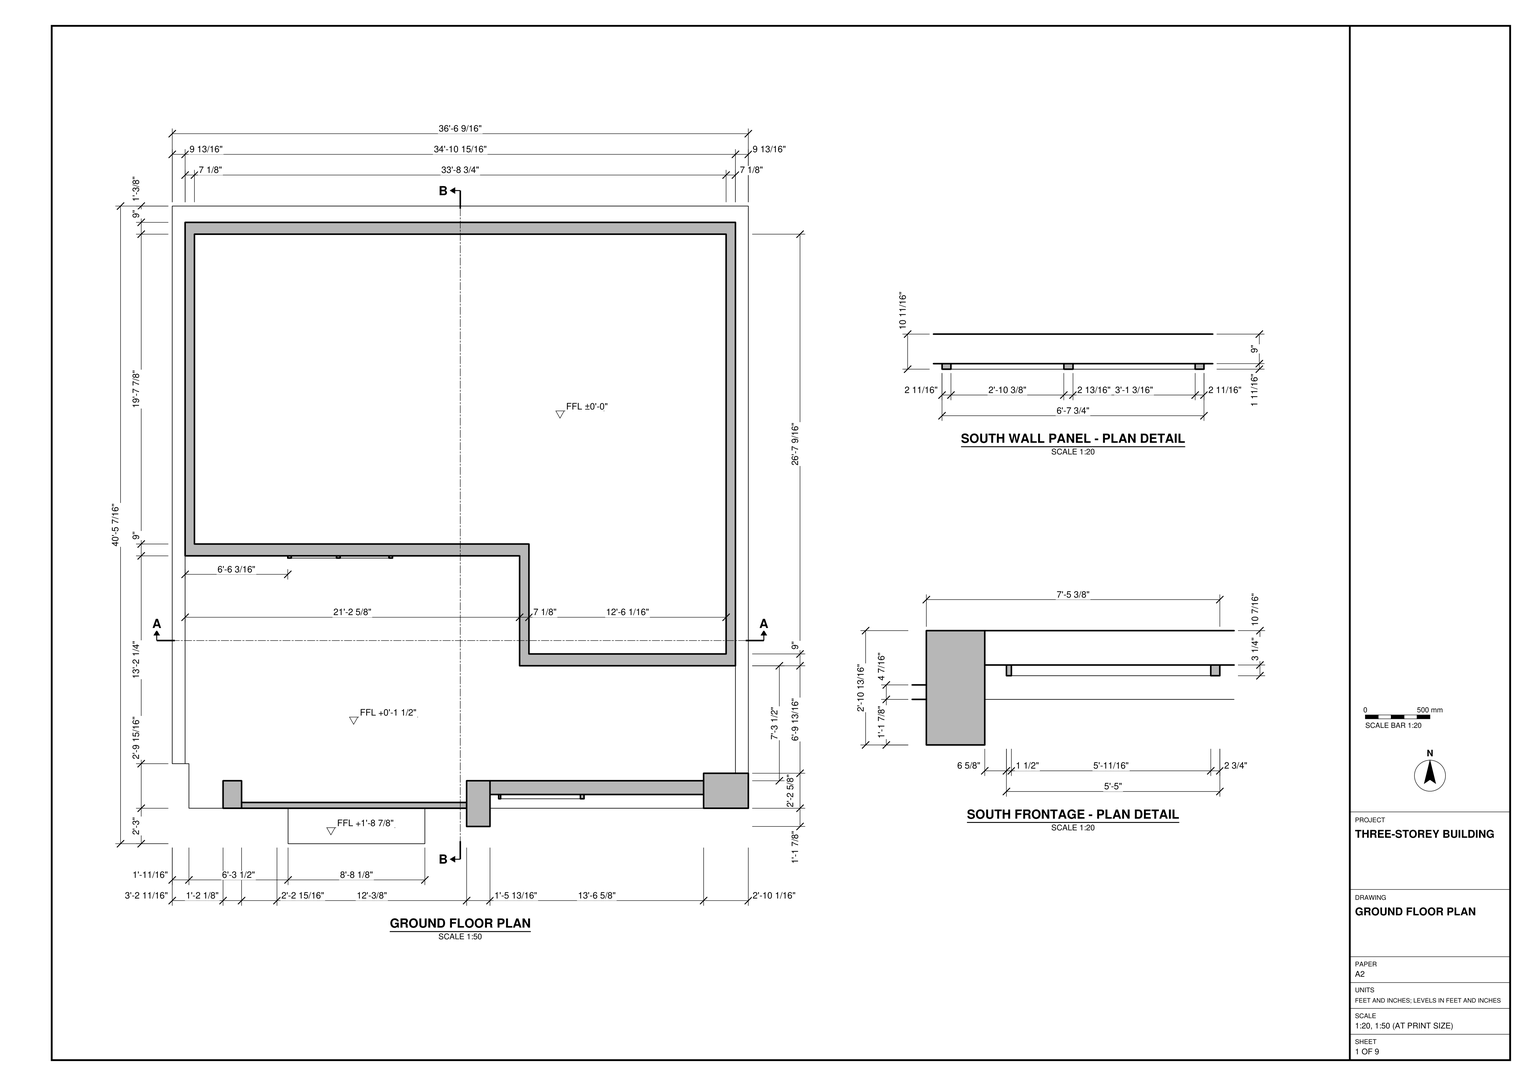
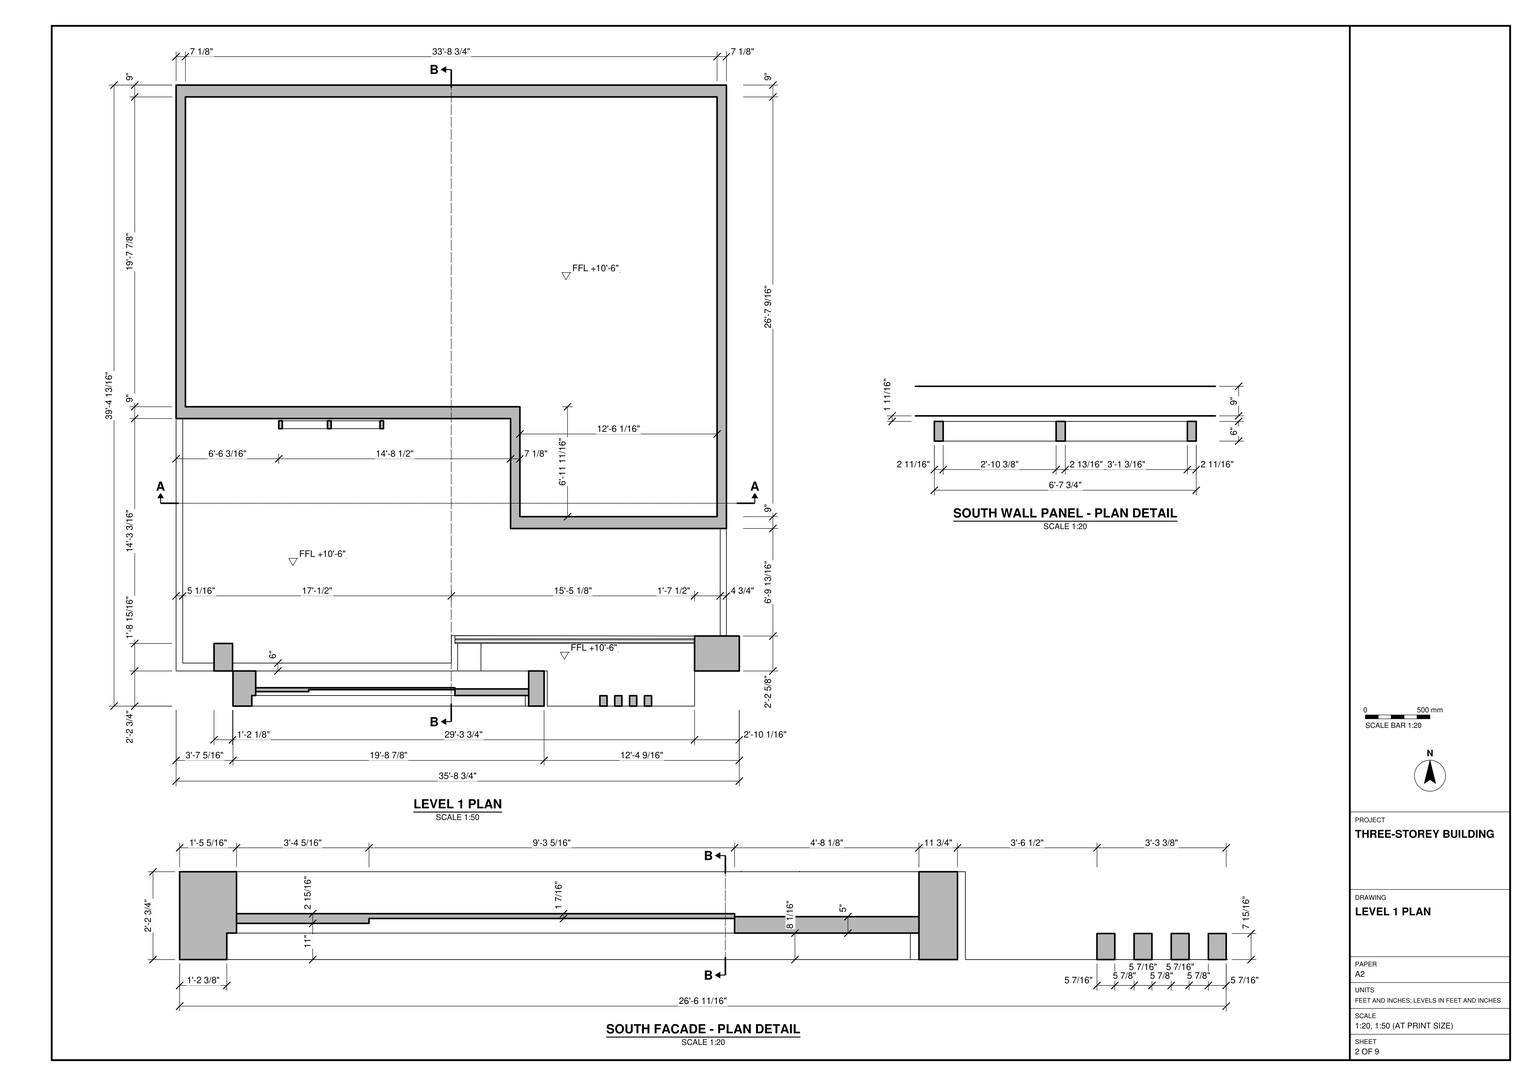
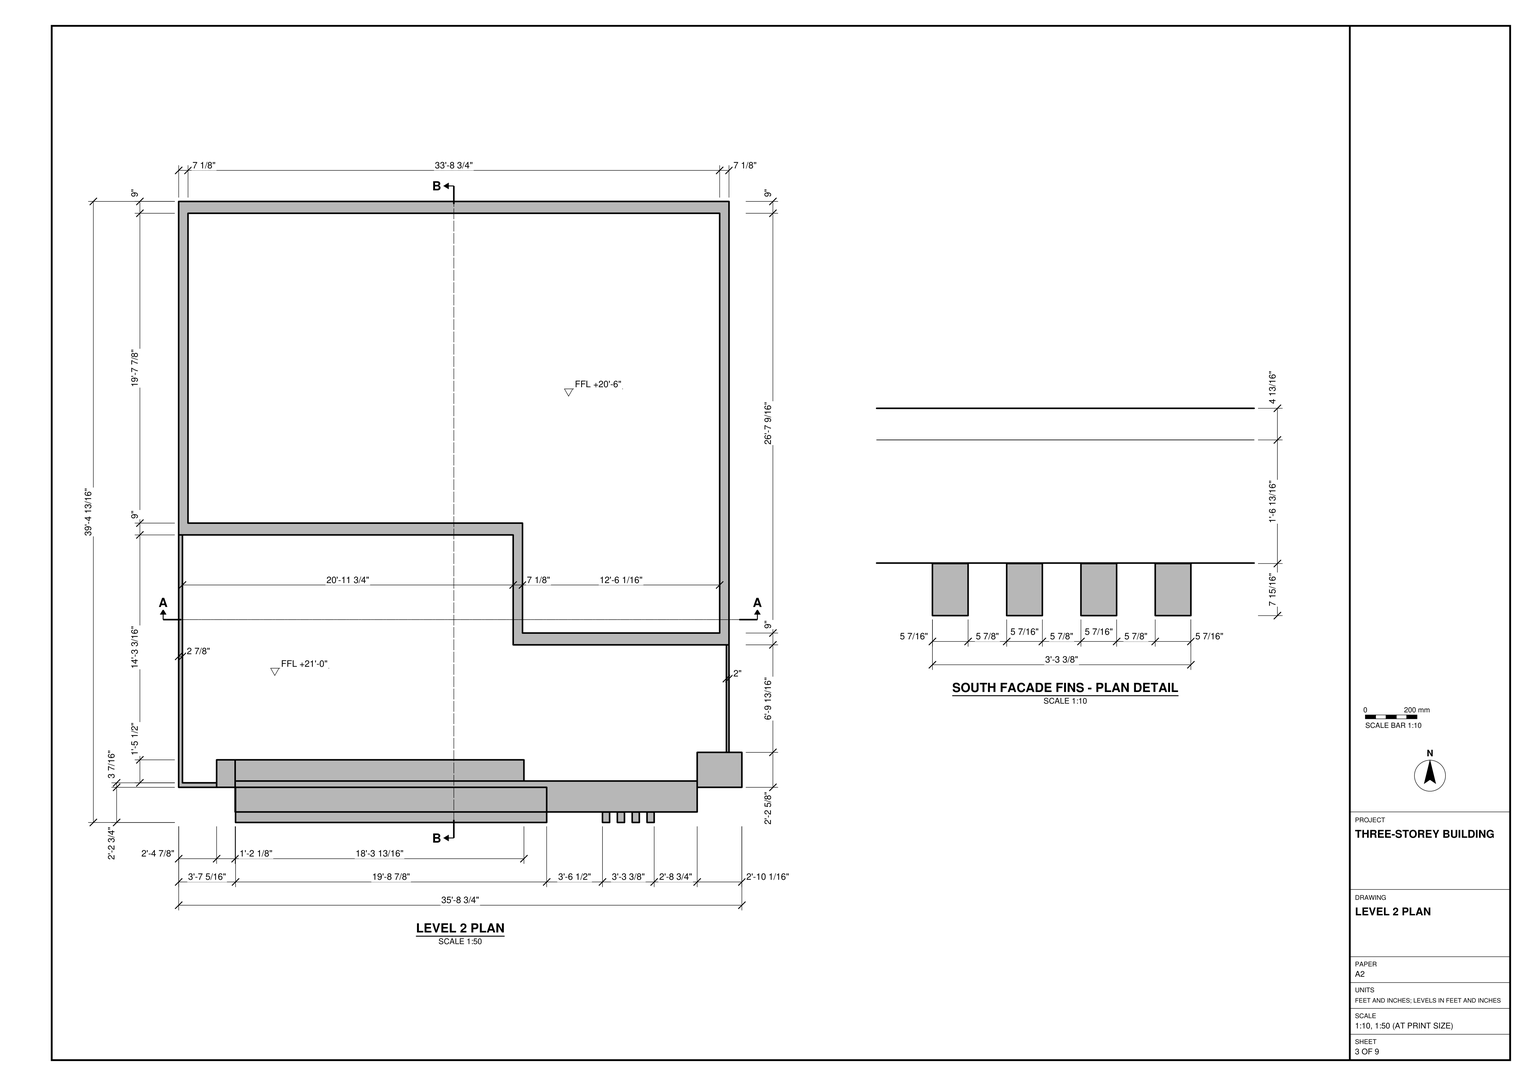
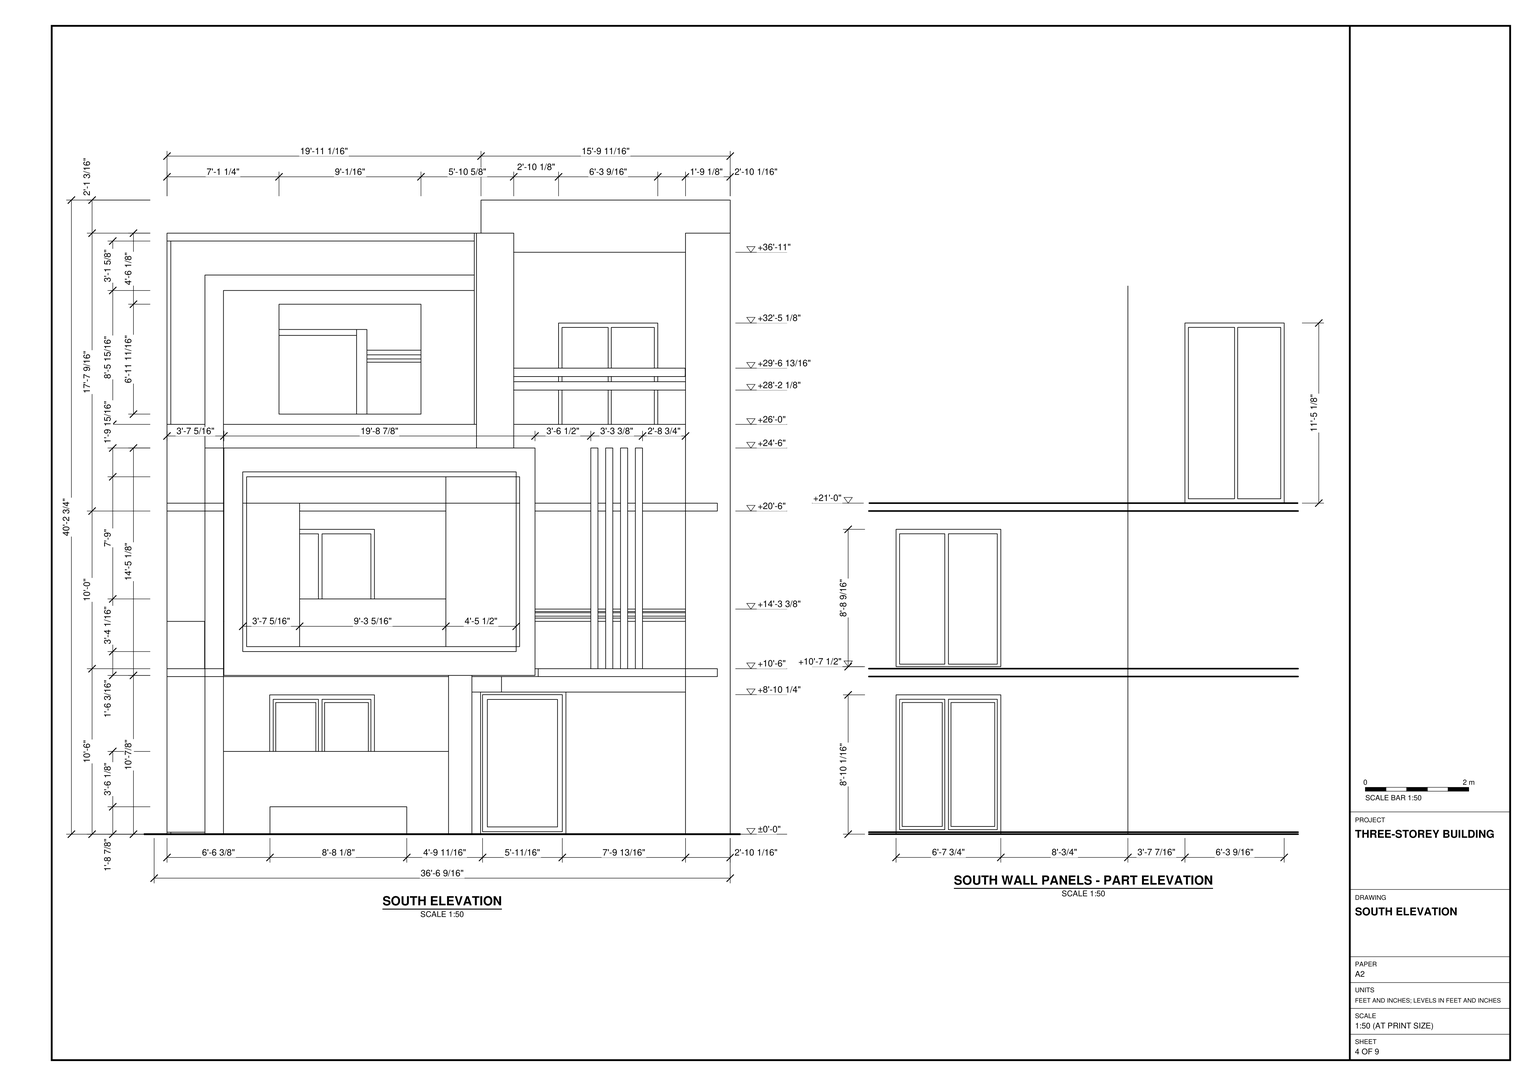
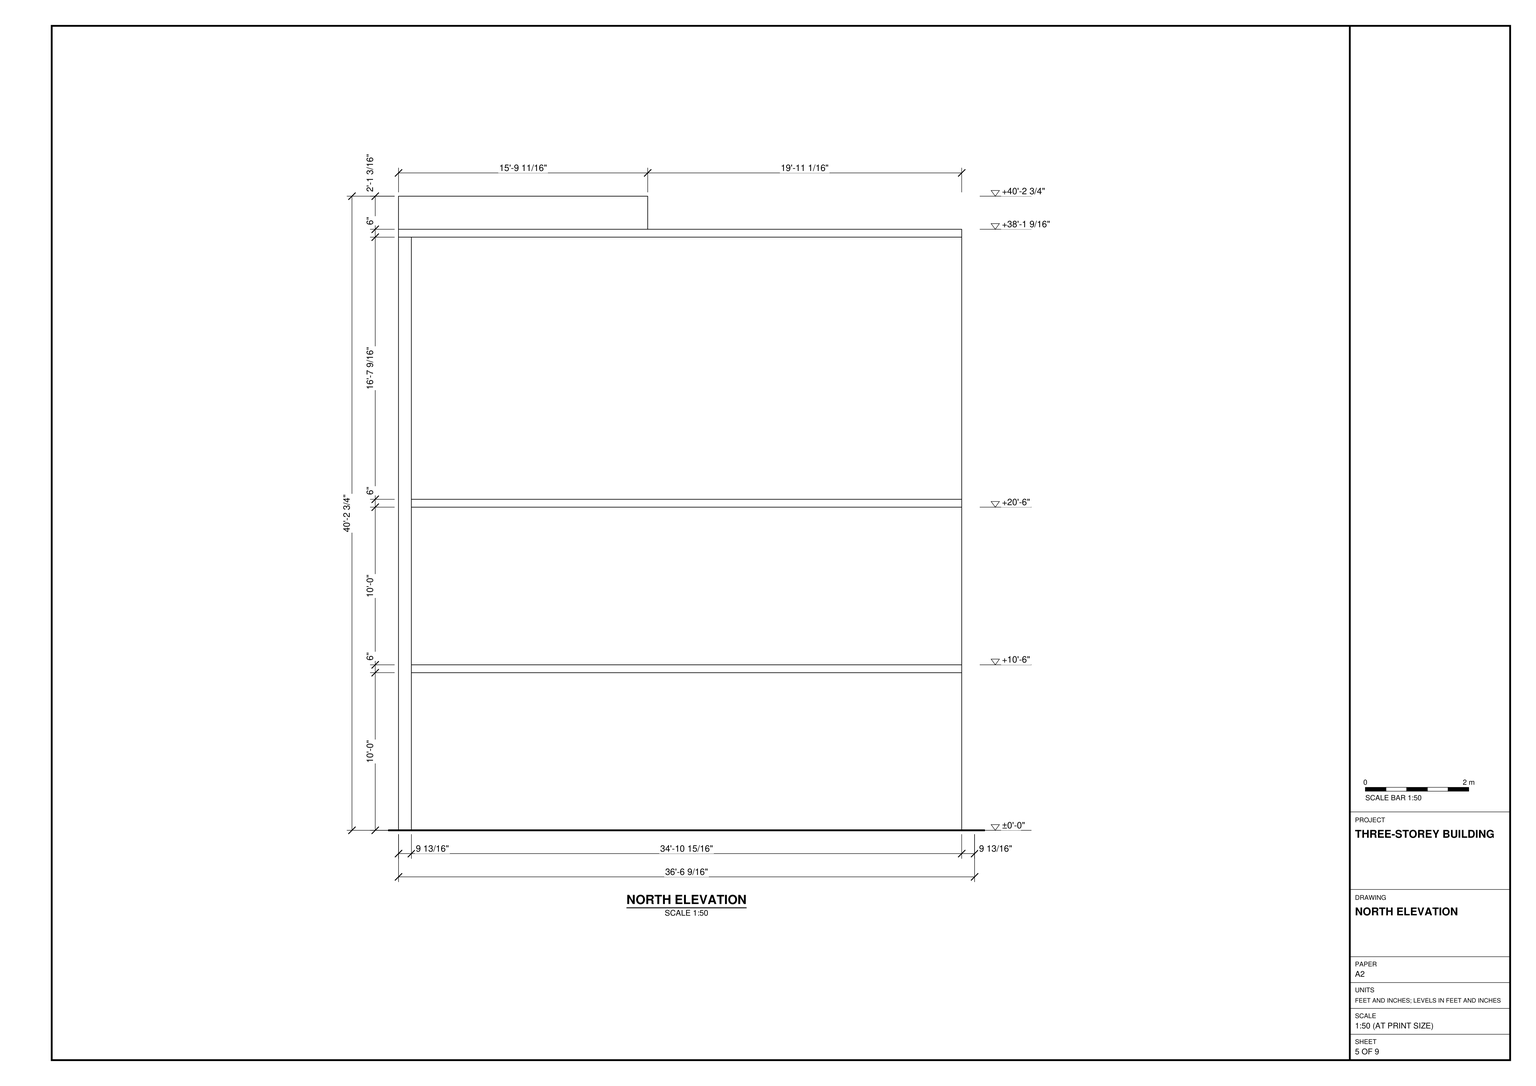
Build the three-storey building in SketchUp from task_files/diagram_01.pdf. Work in feet and inches. Set the overall width along X to 36'-6 9/16", depth along Y to 40'-5 7/16", and height along Z to 40'-2 3/4". Use finished floor levels of ±0'-0", +10'-6", and +20'-6" relative to the ground floor.

Lay out the enclosed part of each storey with a straight north wall and a stepped south wall. The east bay extends farther south than the west bay, leaving a deeper open area in front of the west bay. Use the wall thicknesses dimensioned in plan, including 9" for the east–west walls and 7 1/8" for the north–south returns. Model the floor slabs, the changes in floor height at the frontage, and the roof profile shown in the sections and elevations.

Use the enlarged plans to locate the panels on the recessed south wall and to set out the frontage piers, openings, projecting horizontal members, and closely spaced fins. Follow the drawings for any stairs, built-in joinery, and main furniture rather than adding an interior layout. Keep walls, slabs, the roof, and each furniture or joinery piece in separate groups or components; use components for repeated parts. Any decor or loose items shown may be represented by suitable library components. Save one SketchUp model as output_files/three_storey_building_with_a_stepped_south_frontage.skp.

# SketchUp Ruby script. Lengths in inches.
U = 1.inch
M = Sketchup.active_model
def pt(a) = Geom::Point3d.new(a.map { |v| v * U })
def face(e, loops, mat)
  f = e.add_face(loops[0].map { |a| pt(a) })
  loops[1..].each { |l| e.add_face(l.map { |a| pt(a) }).erase! }
  f.material = f.back_material = mat if mat
  f
end
# faces: each face lists its corners as indices into pts; further lists are holes
def faces(e, pts, list, mat = nil) = list.each { |f| face(e, (f[0].is_a?(Array) ? f : [f]).map { |l| l.map { |i| pts[i] } }, mat) }
# xy, xz, yz: faces in a plane at the given z, y or x. An outline is a flat list of corners, or four numbers for a rectangle; further outlines are holes
def ring(l) = l.size == 4 ? [[l[0], l[1]], [l[2], l[1]], [l[2], l[3]], [l[0], l[3]]] : l.each_slice(2).to_a
def flat(e, list, mat, &to3) = list.each { |f| face(e, (f[0].is_a?(Array) ? f : [f]).map { |l| ring(l).map { |u, v| to3.(u, v) } }, mat) }
def xy(e, z, list, mat = nil) = flat(e, list, mat) { |x, y| [x, y, z] }
def xz(e, y, list, mat = nil) = flat(e, list, mat) { |x, z| [x, y, z] }
def yz(e, x, list, mat = nil) = flat(e, list, mat) { |y, z| [x, y, z] }
def lines(e, pts, list) = list.each { |a, b| e.add_line(pt(pts[a]), pt(pts[b])) }
# prism: a flat outline (further loops are holes) pulled along v
def prism(e, loops, v, mat = nil)
  f = face(e, loops, mat); d = Geom::Vector3d.new(v.map { |x| x * U })
  f.pushpull(f.normal.samedirection?(d) ? d.length : -d.length)
end
def box(e, o, s, mat = nil) = prism(e, [[o, [o[0] + s[0], o[1], o[2]], [o[0] + s[0], o[1] + s[1], o[2]], [o[0], o[1] + s[1], o[2]]]], [0, 0, s[2]], mat)
def at(x, y, z, deg = 0) = Geom::Transformation.translation(pt([x, y, z])) * Geom::Transformation.rotation(ORIGIN, Z_AXIS, deg.degrees)
def axes(o, x, y, z) = Geom::Transformation.new([*x, 0, *y, 0, *z, 0, *pt(o).to_a, 1])
def part(name) = M.definitions.add(name)
# library, detail: a bought-in or finely detailed component or shape, given as its bounding box
def library(name, o, s) = part(name).tap { |d| box(d.entities, o, s) }
def detail(e, o, s) = box(e.add_group.entities, o, s)
def put(e, d, t, mat = nil) = e.add_instance(d, t).tap { |i| i.material = mat if mat }
def group(e, t, mat = nil) = e.add_group.tap { |g| g.transformation = t; g.material = mat if mat }.entities
root = M.entities
g1 = group(root,at(0,0,0))
prism(g1,[[[87.96,211.47,232.0625],[87.96,211.47,127.5],[167.7,211.47,127.5],[167.7,211.47,232.0625]],[[165.02,211.47,129.4],[127.83,211.47,129.4],[127.83,211.47,228.66],[165.02,211.47,228.66]],[[125.05,211.47,228.66],[125.05,211.47,129.4],[90.65,211.47,129.4],[90.65,211.47,228.66]]],[0,6,0])
xy(g1,0,[[88.19,0,192.32,27],[224.11,13.125,241.9,47.9375],[12.71,27,12.71,60.9375,9.8,60.9375,9.8,219.16,87.96,219.16,87.96,217.47,167.7,217.47,167.7,219.16,264.44,219.16,264.44,135.47,428.75,135.47,428.75,53.625,404.52,53.625,404.52,47.9375,224.11,47.9375,224.11,31.41,52.79,31.41,52.79,47.9375,38.69,47.9375,38.69,27],[38.69,27,52.79,47.9375],[52.79,27,79.73,31.41],
  [79.73,27,88.19,31.41],[88.19,27,192.32,31.41],[192.32,27,224.11,31.41],[241.9,27,404.52,27,404.52,37.47,313.48,37.47,313.48,34.22,248.5,34.22,248.5,37.47,241.9,37.47],[248.5,34.22,313.48,37.47],
  [241.9,37.47,404.52,47.9375],[428.75,53.625,438.55,53.625,438.55,485.4375,0,485.4375,0,60.9375,9.8,60.9375,9.8,473.03,428.75,473.03],[[264.44,135.47,264.44,219.16,9.8,219.16,9.8,473.03,428.75,473.03,428.75,135.47],[271.55,144.47,421.64,144.47,421.64,464.03,16.91,464.03,16.91,228.16,271.55,228.16]],[271.55,144.47,421.64,144.47,421.64,464.03,16.91,464.03,16.91,228.16,271.55,228.16],[87.96,217.47,167.7,219.16]])
xy(g1,1.5,[[12.71,27,38.69,27,38.69,47.9375,52.79,47.9375,52.79,31.41,224.11,31.41,224.11,47.9375,404.52,47.9375,404.52,53.625,428.75,53.625,428.75,135.47,264.44,135.47,264.44,219.16,167.7,219.16,167.7,217.47,87.96,217.47,87.96,219.16,9.8,219.16,9.8,60.9375,12.71,60.9375]])
xy(g1,1.9,[[250.01,34.22,310.72,37.47]])
xy(g1,3.4,[[90.65,217.47,125.05,219.16],[127.83,217.47,165.02,219.16]])
xy(g1,20.875,[[88.19,0,192.32,27]])
xy(g1,63,[[52.79,27,224.11,31.41]])
xy(g1,102.66,[[90.65,217.47,125.05,219.16],[127.83,217.47,165.02,219.16]])
xy(g1,106.0625,[[87.96,217.47,167.7,219.16]])
xy(g1,106.22,[[250.01,34.22,310.72,37.47]])
xy(g1,108.1875,[[248.5,34.22,313.48,37.47],[241.9,37.47,404.52,47.9375]])
xy(g1,120,[[292.36,0.25,292.36,27,264.44,27,264.44,47.9375,428.75,47.9375,428.75,27,404.52,27,404.52,0.25],[9.8,27,9.8,219.16,264.44,219.16,264.44,47.9375,224.11,47.9375,224.11,27,79.73,27,79.73,47.9375,26.8125,47.9375,26.8125,60.9375,12.71,60.9375,12.71,27],[12.71,27,26.8125,60.9375],[26.8125,27,79.73,47.9375],[241.9,27,264.44,47.9375],
  [264.44,47.9375,428.75,135.47],[[264.44,135.47,264.44,219.16,9.8,219.16,9.8,473.03,428.75,473.03,428.75,135.47],[271.55,144.47,421.64,144.47,421.64,464.03,16.91,464.03,16.91,228.16,271.55,228.16]]])
xy(g1,126,[[292.36,0.25,332.43,0.25,332.43,8.18,337.86,8.18,337.86,0.25,343.73,0.25,343.73,8.18,349.16,8.18,349.16,0.25,355.04,0.25,355.04,8.18,360.47,8.18,360.47,0.25,366.35,0.25,366.35,8.18,371.78,8.18,371.78,0.25,404.52,0.25,404.52,47.9375,241.9,47.9375,241.9,27,292.36,27],[332.43,0.25,337.86,8.18],[343.73,0.25,349.16,8.18],[355.04,0.25,360.47,8.18],[366.35,0.25,371.78,8.18],
  [224.11,13.125,241.9,47.9375],[9.8,27,9.8,219.16,14.85,219.16,14.85,33,38.46,33,38.46,27],[38.46,27,52.79,27,52.79,33,219.37,33,219.37,53.9375,404.52,53.625,404.52,47.9375,428.75,47.9375,428.75,53.9375,424.01,53.9375,424.01,135.47,264.44,135.47,264.44,219.16,14.85,219.16,14.85,33,38.46,33],[52.79,27,52.79,33,219.37,33,219.37,53.9375,404.52,53.625,404.52,47.9375,224.11,47.9375,224.11,27],[404.52,27,428.75,47.9375],
  [424.01,53.9375,428.75,135.47],[[264.44,135.47,264.44,219.16,9.8,219.16,9.8,473.03,428.75,473.03,428.75,135.47],[271.55,144.47,421.64,144.47,421.64,464.03,16.91,464.03,16.91,228.16,271.55,228.16]],[271.55,144.47,421.64,144.47,421.64,464.03,16.91,464.03,16.91,228.16,271.55,228.16]])
xy(g1,162,[[9.8,27,38.46,27,38.46,33,14.85,33,14.85,219.16,9.8,219.16],[52.79,27,224.11,27,224.11,47.9375,222.08,47.9375,222.08,53.81,297.83,53.81,219.37,53.9375,219.37,33,52.79,33],[222.08,47.9375,222.08,53.81,297.83,53.81,404.52,53.625,404.52,47.9375],[424.01,53.9375,428.75,135.47]])
xy(g1,164.5,[[222.08,47.9375,404.52,47.9375,404.52,53.625,297.83,53.81,222.08,53.81]])
xy(g1,246,[[9.8,27,264.44,60.9375],[264.44,27,428.75,135.47],[9.8,60.9375,264.44,219.16],[[264.44,135.47,264.44,219.16,9.8,219.16,9.8,473.03,428.75,473.03,428.75,135.47],[271.55,144.47,421.64,144.47,421.64,464.03,16.91,464.03,16.91,228.16,271.55,228.16]],[271.55,144.47,421.64,144.47,421.64,464.03,16.91,464.03,16.91,228.16,271.55,228.16]])
xy(g1,252,[[52.79,8.25,404.52,27],[9.8,27,9.8,219.16,12.6875,219.16,12.6875,30.4375,38.69,30.4375,38.69,27],[38.69,27,52.79,27,52.79,47.9375,272.63,47.9375,272.63,31.8125,404.52,31.8125,404.52,27,428.75,27,428.75,53.625,426.77,53.625,426.77,135.47,264.44,135.47,264.44,219.16,12.6875,219.16,12.6875,30.4375,38.69,30.4375],[52.79,27,404.52,31.8125],[426.77,53.625,428.75,135.47],
  [[264.44,135.47,264.44,219.16,9.8,219.16,9.8,473.03,428.75,473.03,428.75,135.47],[271.55,144.47,421.64,144.47,421.64,464.03,16.91,464.03,16.91,228.16,271.55,228.16]]])
xy(g1,294,[[245.41,0.25,269.66,8.25],[269.66,0.25,273.76,8.25],[332.43,0.25,337.86,8.18],[343.73,0.25,349.16,8.18],[355.04,0.25,360.47,8.18],
  [366.35,0.25,371.78,8.18]])
xy(g1,312,[[52.79,8.25,245.41,8.25,243.73,31.8125,52.79,31.8125],[273.76,8.25,404.52,8.25,404.52,31.8125,272.08,31.8125],[9.8,27,38.69,27,38.69,30.4375,12.6875,30.4375,12.6875,219.16,9.8,219.16],[426.77,53.625,428.75,135.47]])
xy(g1,319.8,[[95.0625,31.8125,154.12,47.9375],[154.12,31.8125,161.99,47.9375],[161.99,31.8125,203.14,47.9375]])
xy(g1,358,[[38.69,31.8125,52.79,47.9375]])
xy(g1,379.72,[[95.0625,31.8125,154.12,47.9375]])
xy(g1,384.23,[[95.0625,31.8125,154.12,47.9375],[154.12,31.8125,161.99,47.9375]])
xy(g1,403.46,[[95.0625,31.8125,203.14,47.9375]])
xy(g1,413.92,[[52.79,27,243.73,31.8125]])
xy(g1,425.6875,[[38.69,27,243.73,27,243.73,31.8125,272.63,31.8125,272.63,47.9375,38.69,47.9375]])
xy(g1,443,[[248.84,31.8125,248.84,170.625,260.46,170.625,260.46,42.72,404.52,42.72,404.52,31.8125]])
xy(g1,451.5625,[[404.52,31.8125,426.77,53.625],[426.77,31.8125,428.75,53.625],[428.75,31.8125,438.55,53.625],[260.46,42.72,260.46,135.47,426.77,135.47,426.77,53.625,404.52,53.625,404.52,42.72],[426.77,53.625,428.75,135.47],
  [428.75,53.625,438.55,473.03],[[264.44,135.47,264.44,219.16,9.8,219.16,9.8,473.03,428.75,473.03,428.75,135.47],[271.55,144.47,421.64,144.47,421.64,464.03,16.91,464.03,16.91,228.16,271.55,228.16]],[260.46,135.47,260.46,170.625,248.84,170.625,248.84,219.16,264.44,219.16,264.44,135.47],[9.8,161.41,248.84,219.16]])
xy(g1,457.5625,[[245.41,0.25,273.76,0.25,273.76,8.25,272.08,31.8125,243.73,31.8125,245.41,8.25],[404.52,27,438.55,31.8125],[248.84,41.51,438.55,41.51,438.55,473.03,9.8,473.03,9.8,161.41,248.84,161.41]])
xy(g1,482.75,[[248.84,31.8125,438.55,41.51]])
xz(g1,0,[[88.19,0,192.32,20.875]])
xz(g1,0.25,[[292.36,120,404.52,126],[332.43,126,337.86,294],[343.73,126,349.16,294],[355.04,126,360.47,294],[366.35,126,371.78,294],
  [245.41,294,273.76,457.5625]])
xz(g1,8.18,[[332.43,126,337.86,294],[343.73,126,349.16,294],[355.04,126,360.47,294],[366.35,126,371.78,294]])
xz(g1,8.25,[[52.79,252,404.52,252,404.52,312,273.76,312,273.76,294,245.41,294,245.41,312,52.79,312]])
xz(g1,13.125,[[224.11,0,241.9,126]])
xz(g1,27,[[12.71,0,38.69,1.5],[38.69,0,52.79,120],[52.79,0,88.19,0,88.19,20.875,192.32,20.875,192.32,0,224.11,0,224.11,63,52.79,63],[88.19,0,192.32,20.875],[404.52,0,438.55,0,438.55,457.5625,404.52,457.5625,404.52,252,428.75,252,428.75,246,404.52,246,404.52,126,428.75,126,428.75,120,404.52,120],
  [9.8,120,26.8125,126],[26.8125,120,38.69,126],[38.69,120,52.79,126],[52.79,120,224.11,126],[241.9,120,292.36,126],
  [404.52,120,428.75,126],[9.8,126,38.46,162],[38.69,126,52.79,246],[52.79,126,224.11,162],[9.8,246,38.69,252],
  [38.69,246,52.79,252],[52.79,246,404.52,252],[404.52,246,428.75,252],[9.8,252,38.69,312],[38.69,252,52.79,294],
  [38.69,294,52.79,294,52.79,413.92,243.73,413.92,243.73,425.6875,38.69,425.6875]])
xz(g1,30.4375,[[12.6875,252,38.69,312]])
xz(g1,31.41,[[52.79,0,79.73,1.5],[79.73,0,88.19,1.5],[88.19,0,192.32,1.5],[192.32,0,224.11,1.5],[52.79,1.5,224.11,63]])
xz(g1,31.8125,[[52.79,252,272.63,312],[272.63,252,404.52,312],[[52.79,312,243.73,413.92],[95.0625,319.8,203.14,403.46]],[243.73,312,272.08,425.6875],[272.08,312,272.63,425.6875],
  [154.12,319.8,161.99,384.23],[95.0625,379.72,154.12,384.23],[243.73,425.6875,243.73,457.5625,248.84,457.5625,248.84,443,272.08,443,272.08,425.6875],[248.84,443,272.08,457.5625],[272.08,443,404.52,443,404.52,457.5625,438.55,457.5625,438.55,482.75,248.84,482.75,248.84,457.5625,272.08,457.5625],
  [404.52,451.5625,426.77,457.5625],[426.77,451.5625,428.75,457.5625]])
xz(g1,33,[[14.85,126,38.46,162],[52.79,126,219.37,162]])
xz(g1,34.22,[[[248.5,0,313.48,108.1875],[250.01,1.9,310.72,106.22]]])
xz(g1,37.47,[[241.9,0,248.5,108.1875],[[248.5,0,313.48,108.1875],[250.01,1.9,310.72,106.22]],[313.48,0,404.52,108.1875],[[250.01,1.9,310.72,106.22],[253.65,5.55,307.08,102.58]],[253.65,5.55,307.08,102.58]])
xz(g1,41.51,[[248.84,457.5625,438.55,482.75]])
xz(g1,42.72,[[260.46,443,404.52,451.5625]])
xz(g1,47.9375,[[38.69,0,52.79,1.5],[224.11,0,241.9,1.5],[241.9,0,404.52,1.5],[38.69,1.5,52.79,120],[224.11,1.5,241.9,120],
  [241.9,1.5,404.52,108.1875],[38.69,120,52.79,126],[224.11,120,241.9,126],[241.9,120,428.75,126],[38.69,126,52.79,358],
  [224.11,126,404.52,162],[222.08,162,404.52,164.5],[[52.79,252,52.79,358,38.69,358,38.69,425.6875,272.63,425.6875,272.63,252],[95.0625,319.8,203.14,403.46]],[154.12,319.8,161.99,384.23],[95.0625,379.72,154.12,384.23]])
xz(g1,53.625,[[404.52,0,428.75,1.5],[[428.75,0,428.75,1.5,404.52,1.5,404.52,451.5625,438.55,451.5625,438.55,0],[426.77,252,428.75,312]],[426.77,252,428.75,312]])
xz(g1,53.81,[[222.08,162,297.83,164.5]])
xz(g1,53.9375,[[424.01,126,428.75,162]])
xz(g1,60.9375,[[9.8,0,12.71,1.5]])
xz(g1,135.47,[[264.44,0,428.75,1.5],[264.44,1.5,428.75,120],[264.44,120,428.75,126],[264.44,126,424.01,126,424.01,162,428.75,162,428.75,246,264.44,246],[424.01,126,428.75,162],
  [264.44,246,428.75,252],[264.44,252,307.87,252,307.87,389.125,383.41,389.125,383.41,252,426.77,252,426.77,451.5625,264.44,451.5625],[[307.87,252,383.41,389.125],[310.5,255.33,345.64,385.8],[348.02,255.33,380.78,385.8]],[426.77,252,428.75,312],[310.5,255.33,345.64,385.8],
  [348.02,255.33,380.78,385.8],[426.77,312,428.75,451.5625]])
xz(g1,144.47,[[271.55,0,421.64,120],[271.55,120,421.64,126],[271.55,126,421.64,246],[271.55,246,421.64,252],[271.55,252,421.64,451.5625]])
xz(g1,161.41,[[9.8,451.5625,248.84,457.5625]])
xz(g1,170.625,[[248.84,443,260.46,451.5625]])
xz(g1,217.47,[[87.96,0,167.7,1.5],[[87.96,1.5,167.7,106.0625],[127.83,3.4,165.02,102.66],[90.65,3.4,125.05,102.66]]])
xz(g1,219.16,[[9.8,0,87.96,1.5],[[87.96,0,167.7,106.0625],[127.83,3.4,165.02,102.66],[90.65,3.4,125.05,102.66]],[167.7,0,264.44,1.5],[9.8,1.5,87.96,1.5,87.96,106.0625,167.7,106.0625,167.7,1.5,264.44,1.5,264.44,120,9.8,120],[[90.65,3.4,125.05,102.66],[92.59,5.85,123.11,100.21]],
  [[127.83,3.4,165.02,102.66],[129.77,5.85,163.08,100.21]],[92.59,5.85,123.11,100.21],[129.77,5.85,163.08,100.21],[9.8,120,264.44,126],[14.85,126,264.44,126,264.44,246,9.8,246,9.8,162,14.85,162],
  [9.8,126,14.85,162],[9.8,246,264.44,252],[9.8,252,12.6875,312],[12.6875,252,264.44,451.5625],[9.8,312,12.6875,451.5625]])
xz(g1,228.16,[[16.91,0,271.55,120],[16.91,120,271.55,126],[16.91,126,271.55,246],[16.91,246,271.55,252],[16.91,252,271.55,451.5625]])
xz(g1,464.03,[[16.91,0,421.64,120],[16.91,120,421.64,126],[16.91,126,421.64,246],[16.91,246,421.64,252],[16.91,252,421.64,451.5625]])
xz(g1,473.03,[[9.8,0,428.75,120],[9.8,120,428.75,126],[9.8,126,428.75,246],[9.8,246,428.75,252],[9.8,252,428.75,451.5625],
  [9.8,451.5625,438.55,457.5625]])
yz(g1,9.8,[[60.9375,0,219.16,1.5],[219.16,0,473.03,120],[27,120,219.16,126],[219.16,120,473.03,126],[27,126,219.16,162],
  [219.16,126,473.03,246],[27,246,219.16,252],[219.16,246,473.03,252],[27,252,219.16,312],[219.16,252,473.03,451.5625],
  [161.41,451.5625,473.03,457.5625]])
yz(g1,12.6875,[[30.4375,252,219.16,312]])
yz(g1,12.71,[[27,0,60.9375,1.5]])
yz(g1,14.85,[[33,126,219.16,162]])
yz(g1,16.91,[[228.16,0,464.03,120],[228.16,120,464.03,126],[228.16,126,464.03,246],[228.16,246,464.03,252],[228.16,252,464.03,451.5625]])
yz(g1,38.46,[[27,126,33,162]])
yz(g1,38.69,[[27,0,47.9375,1.5],[27,1.5,27,252,30.4375,252,30.4375,425.6875,31.8125,425.6875,31.8125,358,47.9375,358,47.9375,1.5],[27,252,30.4375,312],[27,312,30.4375,425.6875],[31.8125,358,47.9375,425.6875]])
yz(g1,52.79,[[27,0,31.41,63],[31.41,0,47.9375,1.5],[31.41,1.5,47.9375,1.5,47.9375,126,27,126,27,63,31.41,63],[27,126,33,162],[33,126,47.9375,126,47.9375,252,27,252,27,162,33,162],
  [8.25,252,27,294],[27,252,31.8125,312],[31.8125,252,47.9375,358],[8.25,294,27,312],[27,312,31.8125,413.92]])
yz(g1,87.96,[[217.47,0,219.16,1.5],[217.47,1.5,219.16,106.0625]])
yz(g1,88.19,[[0,0,27,20.875]])
yz(g1,90.65,[[217.47,3.4,219.16,102.66]])
yz(g1,95.0625,[[31.8125,319.8,47.9375,379.72],[31.8125,379.72,47.9375,384.23],[31.8125,384.23,47.9375,403.46]])
yz(g1,125.05,[[217.47,3.4,219.16,102.66]])
yz(g1,127.83,[[217.47,3.4,219.16,102.66]])
yz(g1,154.12,[[31.8125,319.8,47.9375,379.72],[31.8125,379.72,47.9375,384.23]])
yz(g1,161.99,[[[31.8125,319.8,47.9375,384.23],[36.6,364.95,36.15,365.01,35.73,365.18,35.37,365.46,35.09,365.82,34.91,366.24,34.85,366.7,34.91,367.15,35.09,367.57,35.37,367.94,35.73,368.21,36.15,368.39,36.6,368.45,37.06,368.39,37.48,368.21,37.84,367.94,38.12,367.57,38.29,367.15,38.35,366.7,38.29,366.24,38.12,365.82,37.84,365.46,37.48,365.18,37.06,365.01],[36.6,359.31,36.28,359.35,35.98,359.47,35.72,359.67,35.52,359.93,35.4,360.23,35.35,360.56,35.4,360.88,35.52,361.18,35.72,361.44,35.98,361.64,36.28,361.76,36.6,361.81,36.93,361.76,37.23,361.64,37.49,361.44,37.6875,361.18,37.8125,360.88,37.85,360.56,37.8125,360.23,37.6875,359.93,37.49,359.67,37.23,359.47,36.93,359.35]],[36.6,359.31,36.28,359.35,35.98,359.47,35.72,359.67,35.52,359.93,35.4,360.23,35.35,360.56,35.4,360.88,35.52,361.18,35.72,361.44,35.98,361.64,36.28,361.76,36.6,361.81,36.93,361.76,37.23,361.64,37.49,361.44,37.6875,361.18,37.8125,360.88,37.85,360.56,37.8125,360.23,37.6875,359.93,37.49,359.67,37.23,359.47,36.93,359.35],[36.6,364.95,36.15,365.01,35.73,365.18,35.37,365.46,35.09,365.82,34.91,366.24,34.85,366.7,34.91,367.15,35.09,367.57,35.37,367.94,35.73,368.21,36.15,368.39,36.6,368.45,37.06,368.39,37.48,368.21,37.84,367.94,38.12,367.57,38.29,367.15,38.35,366.7,38.29,366.24,38.12,365.82,37.84,365.46,37.48,365.18,37.06,365.01]])
yz(g1,165.02,[[217.47,3.4,219.16,102.66]])
yz(g1,167.7,[[217.47,0,219.16,1.5],[217.47,1.5,219.16,106.0625]])
yz(g1,192.32,[[0,0,27,20.875]])
yz(g1,203.14,[[[31.8125,319.8,47.9375,403.46],[36.6,359.31,36.93,359.35,37.23,359.47,37.49,359.67,37.6875,359.93,37.8125,360.23,37.85,360.56,37.8125,360.88,37.6875,361.18,37.49,361.44,37.23,361.64,36.93,361.76,36.6,361.81,36.28,361.76,35.98,361.64,35.72,361.44,35.52,361.18,35.4,360.88,35.35,360.56,35.4,360.23,35.52,359.93,35.72,359.67,35.98,359.47,36.28,359.35]]])
yz(g1,204.26,[[36.6,364.95,37.06,365.01,37.48,365.18,37.84,365.46,38.12,365.82,38.29,366.24,38.35,366.7,38.29,367.15,38.12,367.57,37.84,367.94,37.48,368.21,37.06,368.39,36.6,368.45,36.15,368.39,35.73,368.21,35.37,367.94,35.09,367.57,34.91,367.15,34.85,366.7,34.91,366.24,35.09,365.82,35.37,365.46,35.73,365.18,36.15,365.01]])
yz(g1,219.37,[[33,126,53.9375,162]])
yz(g1,222.08,[[47.9375,162,53.81,164.5],[50.19,165.98,49.85,166.02,49.54,166.15,49.26,166.36,49.05,166.63,48.92,166.95,48.88,167.29,48.92,167.63,49.05,167.95,49.26,168.22,49.54,168.43,49.85,168.56,50.19,168.6,50.53,168.56,50.85,168.43,51.12,168.22,51.33,167.95,51.46,167.63,51.5,167.29,51.46,166.95,51.33,166.63,51.12,166.36,50.85,166.15,50.53,166.02],[49.67,169.5,49.43,169.54,49.2,169.64,49.02,169.8,48.875,170,48.79,170.22,48.77,170.47,48.81,170.71,48.91,170.93,49.06,171.12,49.26,171.26,49.49,171.35,49.74,171.37,49.98,171.33,50.2,171.23,50.39,171.07,50.53,170.87,50.62,170.64,50.64,170.4,50.6,170.16,50.5,169.9375,50.34,169.75,50.14,169.61,49.91,169.52]])
yz(g1,224.11,[[13.125,0,13.125,126,27,126,27,120,47.9375,120,47.9375,63,27,63,27,0],[27,0,31.41,22.45],[31.41,0,47.9375,1.5],[31.41,1.5,47.9375,22.45],[27,22.45,31.41,31.5],
  [31.41,22.45,47.9375,31.5],[27,31.5,31.41,63],[31.41,31.5,47.9375,63],[27,120,47.9375,126],[27,126,47.9375,162]])
yz(g1,241.9,[[13.125,0,37.47,0,37.47,120,27,120,27,126,13.125,126],[37.47,0,47.9375,108.1875],[37.47,108.1875,47.9375,120],[27,120,37.47,126],[37.47,120,47.9375,126]])
yz(g1,243.73,[[27,413.92,31.8125,425.6875]])
yz(g1,245.41,[[0.25,294,8.25,457.5625]])
yz(g1,248.5,[[34.22,0,37.47,108.1875]])
yz(g1,248.84,[[31.8125,443,161.41,457.5625],[161.41,443,170.625,451.5625],[31.8125,457.5625,41.51,482.75]])
yz(g1,250.01,[[34.22,1.9,37.47,106.22]])
yz(g1,260.46,[[42.72,443,135.47,451.5625],[135.47,443,170.625,451.5625]])
yz(g1,264.44,[[135.47,0,219.16,1.5],[135.47,1.5,219.16,120],[135.47,120,219.16,126],[135.47,126,219.16,246],[135.47,246,219.16,252],
  [135.47,252,219.16,451.5625]])
yz(g1,271.55,[[144.47,0,228.16,120],[144.47,120,228.16,126],[144.47,126,228.16,246],[144.47,246,228.16,252],[144.47,252,228.16,451.5625]])
yz(g1,272.63,[[31.8125,252,47.9375,425.6875]])
yz(g1,273.76,[[0.25,294,8.25,457.5625]])
yz(g1,292.36,[[0.25,120,27,126]])
yz(g1,310.72,[[34.22,1.9,37.47,106.22]])
yz(g1,313.48,[[34.22,0,37.47,108.1875]])
yz(g1,332.43,[[0.25,126,8.18,294]])
yz(g1,337.86,[[0.25,126,8.18,294]])
yz(g1,343.73,[[0.25,126,8.18,294]])
yz(g1,349.16,[[0.25,126,8.18,294]])
yz(g1,355.04,[[0.25,126,8.18,294]])
yz(g1,360.47,[[0.25,126,8.18,294]])
yz(g1,366.35,[[0.25,126,8.18,294]])
yz(g1,371.78,[[0.25,126,8.18,294]])
yz(g1,404.52,[[27,0,27,126,53.625,126,53.625,1.5,47.9375,1.5,47.9375,108.1875,37.47,108.1875,37.47,0],[37.47,0,47.9375,108.1875],[47.9375,0,53.625,1.5],[0.25,120,27,126],[[27,126,27,252,31.8125,252,31.8125,312,27,312,27,457.5625,31.8125,457.5625,31.8125,443,42.72,443,42.72,451.5625,53.625,451.5625,53.625,164.5,47.9375,164.5,47.9375,126],[50.19,165.98,50.53,166.02,50.85,166.15,51.12,166.36,51.33,166.63,51.46,166.95,51.5,167.29,51.46,167.63,51.33,167.95,51.12,168.22,50.85,168.43,50.53,168.56,50.19,168.6,49.85,168.56,49.54,168.43,49.26,168.22,49.05,167.95,48.92,167.63,48.88,167.29,48.92,166.95,49.05,166.63,49.26,166.36,49.54,166.15,49.85,166.02],[49.67,169.5,49.91,169.52,50.14,169.61,50.34,169.75,50.5,169.9375,50.6,170.16,50.64,170.4,50.62,170.64,50.53,170.87,50.39,171.07,50.2,171.23,49.98,171.33,49.74,171.37,49.49,171.35,49.26,171.26,49.06,171.12,48.91,170.93,48.81,170.71,48.77,170.47,48.79,170.22,48.875,170,49.02,169.8,49.2,169.64,49.43,169.54]],
  [47.9375,126,53.625,162],[47.9375,162,53.625,164.5],[50.19,165.98,50.53,166.02,50.85,166.15,51.12,166.36,51.33,166.63,51.46,166.95,51.5,167.29,51.46,167.63,51.33,167.95,51.12,168.22,50.85,168.43,50.53,168.56,50.19,168.6,49.85,168.56,49.54,168.43,49.26,168.22,49.05,167.95,48.92,167.63,48.88,167.29,48.92,166.95,49.05,166.63,49.26,166.36,49.54,166.15,49.85,166.02],[49.67,169.5,49.91,169.52,50.14,169.61,50.34,169.75,50.5,169.9375,50.6,170.16,50.64,170.4,50.62,170.64,50.53,170.87,50.39,171.07,50.2,171.23,49.98,171.33,49.74,171.37,49.49,171.35,49.26,171.26,49.06,171.12,48.91,170.93,48.81,170.71,48.77,170.47,48.79,170.22,48.875,170,49.02,169.8,49.2,169.64,49.43,169.54],[8.25,252,27,312],
  [27,252,31.8125,312],[31.8125,443,42.72,451.5625]])
yz(g1,421.64,[[144.47,0,464.03,120],[144.47,120,464.03,126],[144.47,126,208.85,246],[208.85,126,222.91,246],[222.91,126,464.03,246],
  [144.47,246,464.03,252],[144.47,252,464.03,451.5625]])
yz(g1,424.01,[[53.9375,126,135.47,162]])
yz(g1,426.77,[[53.625,252,135.47,312]])
yz(g1,428.75,[[53.625,0,135.47,1.5],[135.47,0,473.03,120],[27,120,47.9375,126],[47.9375,120,53.625,126],[53.625,120,135.47,126],
  [135.47,120,473.03,126],[53.9375,126,135.47,162],[135.47,126,473.03,246],[27,246,53.625,252],[53.625,246,135.47,252],
  [135.47,246,473.03,252],[53.625,252,135.47,312],[135.47,252,473.03,451.5625]])
yz(g1,438.55,[[27,0,53.625,451.5625],[27,451.5625,473.03,451.5625,473.03,457.5625,41.51,457.5625,41.51,482.75,31.8125,482.75,31.8125,457.5625,27,457.5625]])
# 20 loose lines left out
p = [[404.52,53.625,126],[219.37,53.9375,126],[219.37,53.9375,162],[297.83,53.81,162],[404.52,53.625,162],[297.83,53.81,164.5],
  [404.52,53.625,164.5],[404.52,49.85,166.02],[404.52,49.54,166.15],[222.08,49.54,166.15],[222.08,49.85,166.02],[404.52,50.19,165.98],
  [222.08,50.19,165.98],[404.52,50.53,166.02],[222.08,50.53,166.02],[404.52,50.85,166.15],[222.08,50.85,166.15],[404.52,49.26,166.36],
  [222.08,49.26,166.36],[404.52,51.12,166.36],[222.08,51.12,166.36],[404.52,49.05,166.63],[222.08,49.05,166.63],[404.52,51.33,166.63],
  [222.08,51.33,166.63],[404.52,48.92,166.95],[222.08,48.92,166.95],[404.52,51.46,166.95],[222.08,51.46,166.95],[404.52,48.88,167.29],
  [222.08,48.88,167.29],[404.52,51.5,167.29],[222.08,51.5,167.29],[404.52,48.92,167.63],[222.08,48.92,167.63],[404.52,51.46,167.63],
  [222.08,51.46,167.63],[404.52,49.05,167.95],[222.08,49.05,167.95],[404.52,51.33,167.95],[222.08,51.33,167.95],[404.52,49.26,168.22],
  [222.08,49.26,168.22],[404.52,51.12,168.22],[222.08,51.12,168.22],[404.52,49.54,168.43],[222.08,49.54,168.43],[404.52,50.85,168.43],
  [222.08,50.85,168.43],[404.52,49.85,168.56],[222.08,49.85,168.56],[404.52,50.53,168.56],[222.08,50.53,168.56],[404.52,50.19,168.6],
  [222.08,50.19,168.6],[404.52,49.43,169.54],[404.52,49.2,169.64],[222.08,49.2,169.64],[222.08,49.43,169.54],[404.52,49.67,169.5],
  [222.08,49.67,169.5],[404.52,49.91,169.52],[222.08,49.91,169.52],[404.52,50.14,169.61],[222.08,50.14,169.61],[404.52,49.02,169.8],
  [222.08,49.02,169.8],[404.52,50.34,169.75],[222.08,50.34,169.75],[404.52,50.5,169.9375],[222.08,50.5,169.9375],[404.52,48.875,170],
  [222.08,48.875,170],[404.52,50.6,170.16],[222.08,50.6,170.16],[404.52,48.79,170.22],[222.08,48.79,170.22],[404.52,48.77,170.47],
  [222.08,48.77,170.47],[404.52,50.64,170.4],[222.08,50.64,170.4],[404.52,50.62,170.64],[222.08,50.62,170.64],[404.52,48.81,170.71],
  [222.08,48.81,170.71],[404.52,50.53,170.87],[222.08,50.53,170.87],[404.52,48.91,170.93],[222.08,48.91,170.93],[404.52,49.06,171.12],
  [222.08,49.06,171.12],[404.52,50.39,171.07],[222.08,50.39,171.07],[404.52,49.26,171.26],[222.08,49.26,171.26],[404.52,50.2,171.23],
  [222.08,50.2,171.23],[404.52,49.98,171.33],[222.08,49.98,171.33],[404.52,49.49,171.35],[222.08,49.49,171.35],[404.52,49.74,171.37],
  [222.08,49.74,171.37],[243.73,31.8125,312],[245.41,8.25,312],[245.41,8.25,457.5625],[243.73,31.8125,457.5625],[243.73,31.8125,425.6875],
  [243.73,31.8125,413.92],[273.76,8.25,312],[272.08,31.8125,312],[272.08,31.8125,425.6875],[272.08,31.8125,443],[272.08,31.8125,457.5625],
  [273.76,8.25,457.5625],[272.83,21.22,352.42],[272.83,21.33,351.6],[272.83,21.22,350.77],[272.86,20.9,350],[272.89,20.4,349.34],
  [272.94,19.74,348.84],[272.99,18.97,348.52],[273.05,18.15,348.41],[273.11,17.33,348.52],[273.17,16.56,348.84],[273.21,15.91,349.34],
  [273.25,15.4,350],[273.27,15.09,350.77],[273.28,14.98,351.6],[273.27,15.09,352.42],[273.25,15.4,353.19],[273.21,15.91,353.85],
  [273.17,16.56,354.36],[273.11,17.33,354.68],[273.05,18.15,354.78],[272.99,18.97,354.68],[272.94,19.74,354.36],[272.89,20.4,353.85],
  [272.86,20.9,353.19],[272.83,21.22,342.11],[272.83,21.33,341.28],[272.83,21.22,340.46],[272.86,20.9,339.69],[272.89,20.4,339.03],
  [272.94,19.74,338.52],[272.99,18.97,338.21],[273.05,18.15,338.1],[273.11,17.33,338.21],[273.17,16.56,338.52],[273.21,15.91,339.03],
  [273.25,15.4,339.69],[273.27,15.09,340.46],[273.28,14.98,341.28],[273.27,15.09,342.11],[273.25,15.4,342.88],[273.21,15.91,343.54],
  [273.17,16.56,344.04],[273.11,17.33,344.36],[273.05,18.15,344.47],[272.99,18.97,344.36],[272.94,19.74,344.04],[272.89,20.4,343.54],
  [272.86,20.9,342.88],[272.83,21.22,331.8],[272.83,21.33,330.97],[272.83,21.22,330.15],[272.86,20.9,329.38],[272.89,20.4,328.72],
  [272.94,19.74,328.21],[272.99,18.97,327.89],[273.05,18.15,327.78],[273.11,17.33,327.89],[273.17,16.56,328.21],[273.21,15.91,328.72],
  [273.25,15.4,329.38],[273.27,15.09,330.15],[273.28,14.98,330.97],[273.27,15.09,331.8],[273.25,15.4,332.57],[273.21,15.91,333.23],
  [273.17,16.56,333.73],[273.11,17.33,334.05],[273.05,18.15,334.16],[272.99,18.97,334.05],[272.94,19.74,333.73],[272.89,20.4,333.23],
  [272.86,20.9,332.57],[407.89,33.55,338.1],[407.95,32.72,338.21],[407.83,34.37,338.21],[407.67,36.72,341.28],[407.67,36.61,342.11],
  [407.7,36.29,342.88],[407.73,35.79,343.54],[407.78,35.13,344.04],[407.83,34.37,344.36],[407.89,33.55,344.47],[407.95,32.72,344.36],
  [408,31.96,344.04],[408.05,31.3,343.54],[408.09,30.8,342.88],[408.11,30.48,342.11],[408.12,30.37,341.28],[408.11,30.48,340.46],
  [408.09,30.8,339.69],[408.05,31.3,339.03],[408,31.96,338.52],[407.78,35.13,338.52],[407.73,35.79,339.03],[407.7,36.29,339.69],
  [407.67,36.61,340.46],[404.08,33.11,348.41],[404.14,32.29,348.52],[404.02,33.93,348.52],[403.85,36.28,351.6],[403.86,36.18,352.42],
  [403.88,35.86,353.19],[403.92,35.35,353.85],[403.97,34.7,354.36],[404.02,33.93,354.68],[404.08,33.11,354.78],[404.14,32.29,354.68],
  [404.19,31.52,354.36],[404.24,30.87,353.85],[404.28,30.36,353.19],[404.3,30.04,352.42],[404.31,29.94,351.6],[404.3,30.04,350.77],
  [404.28,30.36,350],[404.24,30.87,349.34],[404.19,31.52,348.84],[403.97,34.7,348.84],[403.92,35.35,349.34],[403.88,35.86,350],
  [403.86,36.18,350.77],[161.99,35.98,359.47],[161.99,36.28,359.35],[203.14,36.28,359.35],[203.14,35.98,359.47],[161.99,36.6,359.31],
  [203.14,36.6,359.31],[161.99,36.93,359.35],[203.14,36.93,359.35],[161.99,37.23,359.47],[203.14,37.23,359.47],[161.99,35.72,359.67],
  [203.14,35.72,359.67],[161.99,37.49,359.67],[203.14,37.49,359.67],[161.99,35.52,359.93],[203.14,35.52,359.93],[161.99,37.6875,359.93],
  [203.14,37.6875,359.93],[161.99,35.4,360.23],[203.14,35.4,360.23],[161.99,37.8125,360.23],[203.14,37.8125,360.23],[161.99,35.35,360.56],
  [203.14,35.35,360.56],[161.99,37.85,360.56],[203.14,37.85,360.56],[161.99,35.4,360.88],[203.14,35.4,360.88],[161.99,37.8125,360.88],
  [203.14,37.8125,360.88],[161.99,35.52,361.18],[203.14,35.52,361.18],[161.99,37.6875,361.18],[203.14,37.6875,361.18],[161.99,35.72,361.44],
  [203.14,35.72,361.44],[161.99,37.49,361.44],[203.14,37.49,361.44],[161.99,35.98,361.64],[203.14,35.98,361.64],[161.99,37.23,361.64],
  [203.14,37.23,361.64],[161.99,36.28,361.76],[203.14,36.28,361.76],[161.99,36.93,361.76],[203.14,36.93,361.76],[161.99,36.6,361.81],
  [203.14,36.6,361.81],[161.99,36.15,365.01],[161.99,36.6,364.95],[204.26,36.6,364.95],[204.26,36.15,365.01],[161.99,37.06,365.01],
  [204.26,37.06,365.01],[161.99,35.73,365.18],[204.26,35.73,365.18],[161.99,37.48,365.18],[204.26,37.48,365.18],[161.99,35.37,365.46],
  [204.26,35.37,365.46],[161.99,37.84,365.46],[204.26,37.84,365.46],[161.99,35.09,365.82],[204.26,35.09,365.82],[161.99,38.12,365.82],
  [204.26,38.12,365.82],[161.99,34.91,366.24],[204.26,34.91,366.24],[161.99,38.29,366.24],[204.26,38.29,366.24],[161.99,34.85,366.7],
  [204.26,34.85,366.7],[161.99,38.35,366.7],[204.26,38.35,366.7],[161.99,34.91,367.15],[204.26,34.91,367.15],[161.99,38.29,367.15],
  [204.26,38.29,367.15],[161.99,35.09,367.57],[204.26,35.09,367.57],[161.99,38.12,367.57],[204.26,38.12,367.57],[161.99,35.37,367.94],
  [204.26,35.37,367.94],[161.99,37.84,367.94],[204.26,37.84,367.94],[161.99,35.73,368.21],[204.26,35.73,368.21],[161.99,37.48,368.21],
  [204.26,37.48,368.21],[161.99,36.15,368.39],[204.26,36.15,368.39],[161.99,37.06,368.39],[204.26,37.06,368.39],[161.99,36.6,368.45],
  [204.26,36.6,368.45]]
faces(g1,p,[[0,1,2,3,4],[4,3,5,6],[7,8,9,10],[11,7,10,12],[13,11,12,14],[15,13,14,16],[8,17,18,9],[19,15,16,20],
  [17,21,22,18],[23,19,20,24],[21,25,26,22],[27,23,24,28],[25,29,30,26],[31,27,28,32],[29,33,34,30],[35,31,32,36],
  [33,37,38,34],[39,35,36,40],[37,41,42,38],[43,39,40,44],[41,45,46,42],[47,43,44,48],[45,49,50,46],[51,47,48,52],
  [49,53,54,50],[53,51,52,54],[55,56,57,58],[59,55,58,60],[61,59,60,62],[63,61,62,64],[56,65,66,57],[67,63,64,68],
  [69,67,68,70],[65,71,72,66],[73,69,70,74],[71,75,76,72],[75,77,78,76],[79,73,74,80],[81,79,80,82],[77,83,84,78],
  [85,81,82,86],[83,87,88,84],[87,89,90,88],[91,85,86,92],[89,93,94,90],[95,91,92,96],[97,95,96,98],[93,99,100,94],
  [99,101,102,100],[101,97,98,102],[103,104,105,106,107,108],[[109,110,111,112,113,114],[115,116,117,118,119,120,121,122,123,124,125,126,127,128,129,130,131,132,133,134,135,136,137,138],[139,140,141,142,143,144,145,146,147,148,149,150,151,152,153,154,155,156,157,158,159,160,161,162],[163,164,165,166,167,168,169,170,171,172,173,174,175,176,177,178,179,180,181,182,183,184,185,186]],[164,163,186,185,184,183,182,181,180,179,178,177,176,175,174,173,172,171,170,169,168,167,166,165],[139,140,141,142,143,144,145,146,147,148,149,150,151,152,153,154,155,156,157,158,159,160,161,162],[147,146,187,188],[146,145,189,187],
  [190,191,192,193,194,195,196,197,198,199,200,201,202,203,204,205,206,188,187,189,207,208,209,210],[148,147,188,206],[145,144,207,189],[149,148,206,205],[144,143,208,207],[150,149,205,204],[143,142,209,208],[151,150,204,203],
  [142,141,210,209],[152,151,203,202],[141,140,190,210],[153,152,202,201],[140,139,191,190],[154,153,201,200],[139,162,192,191],[155,154,200,199],
  [162,161,193,192],[156,155,199,198],[161,160,194,193],[157,156,198,197],[160,159,195,194],[158,157,197,196],[159,158,196,195],[115,116,117,118,119,120,121,122,123,124,125,126,127,128,129,130,131,132,133,134,135,136,137,138],
  [123,122,211,212],[122,121,213,211],[214,215,216,217,218,219,220,221,222,223,224,225,226,227,228,229,230,212,211,213,231,232,233,234],[124,123,212,230],[121,120,231,213],[125,124,230,229],[120,119,232,231],[126,125,229,228],
  [119,118,233,232],[127,126,228,227],[118,117,234,233],[128,127,227,226],[117,116,214,234],[129,128,226,225],[116,115,215,214],[130,129,225,224],
  [115,138,216,215],[131,130,224,223],[138,137,217,216],[132,131,223,222],[137,136,218,217],[133,132,222,221],[136,135,219,218],[134,133,221,220],
  [135,134,220,219],[235,236,237,238],[236,239,240,237],[239,241,242,240],[241,243,244,242],[245,235,238,246],[243,247,248,244],[249,245,246,250],
  [247,251,252,248],[253,249,250,254],[251,255,256,252],[257,253,254,258],[255,259,260,256],[261,257,258,262],[259,263,264,260],[265,261,262,266],
  [263,267,268,264],[269,265,266,270],[267,271,272,268],[273,269,270,274],[271,275,276,272],[277,273,274,278],[275,279,280,276],[281,277,278,282],
  [279,281,282,280],[283,284,285,286],[284,287,288,285],[289,283,286,290],[287,291,292,288],[293,289,290,294],[291,295,296,292],[297,293,294,298],
  [295,299,300,296],[301,297,298,302],[299,303,304,300],[305,301,302,306],[303,307,308,304],[309,305,306,310],[307,311,312,308],[313,309,310,314],
  [311,315,316,312],[317,313,314,318],[315,319,320,316],[321,317,318,322],[319,323,324,320],[325,321,322,326],[323,327,328,324],[329,325,326,330],
  [327,329,330,328]])
g2 = group(g1,at(53.1,27,120.875))
xy(g2,0,[[0,-26.75,236.85,0]])
xy(g2,18.17,[[14.35,-26.75,222.5,-18.6875]])
xy(g2,21.92,[[222.5,-26.75,225.12,-18.6875],[17.3125,-18.6875,168.98,-18.6875,168.98,-14.23,57.65,-14.23,57.65,-15.73,17.3125,-15.73],[168.98,-18.6875,225.12,-13.68],[17.3125,-15.73,57.65,-15.73,57.65,-14.23,68.17,-14.23,68.17,-12.77,17.3125,-12.77],[68.17,-14.23,168.98,-12.77],
  [168.98,-13.68,225.12,-13.68,225.12,0,17.3125,0,17.3125,-12.77,168.98,-12.77]])
xy(g2,58.23,[[57.65,-14.23,168.98,-12.77]])
xy(g2,151.21,[[222.5,-26.75,225.12,-18.6875],[17.3125,-18.6875,68.17,-15.73],[68.17,-18.6875,68.17,-15.73,57.65,-15.73,57.65,-12.77,17.3125,-12.77,17.3125,0,225.12,0,225.12,-13.68,168.98,-13.68,168.98,-18.6875],[168.98,-18.6875,225.12,-13.68],[17.3125,-15.73,57.65,-12.77]])
xy(g2,154.96,[[14.35,-26.75,222.5,-18.6875]])
xy(g2,173.125,[[0,-26.75,236.85,0]])
xz(g2,-26.75,[[[0,0,236.85,173.125],[14.35,18.17,14.35,154.96,222.5,154.96,222.5,151.21,225.12,151.21,225.12,21.92,222.5,21.92,222.5,18.17]]])
xz(g2,-18.6875,[[14.35,18.17,222.5,18.17,222.5,21.92,17.3125,21.92,17.3125,151.21,222.5,151.21,222.5,154.96,14.35,154.96],[168.98,21.92,222.5,151.21],[222.5,21.92,225.12,151.21]])
xz(g2,-15.73,[[17.3125,21.92,57.65,151.21]])
xz(g2,-14.23,[[57.65,21.92,168.98,58.23]])
xz(g2,-13.68,[[168.98,21.92,225.12,151.21]])
xz(g2,-12.77,[[17.3125,21.92,17.3125,151.21,57.65,151.21,57.65,58.23,168.98,58.23,168.98,21.92]])
xz(g2,0,[[[0,0,236.85,173.125],[17.3125,21.92,225.12,151.21]]])
yz(g2,0,[[-26.75,0,0,173.125]])
yz(g2,14.35,[[-26.75,18.17,-18.6875,154.96]])
yz(g2,17.3125,[[-18.6875,21.92,-15.73,151.21],[-15.73,21.92,-12.77,151.21],[-12.77,21.92,0,151.21]])
yz(g2,57.65,[[-15.73,21.92,-14.23,21.92,-14.23,58.23,-12.77,58.23,-12.77,151.21,-15.73,151.21]])
yz(g2,168.98,[[-18.6875,21.92,-18.6875,151.21,-13.68,151.21,-13.68,58.23,-14.23,58.23,-14.23,21.92],[-14.23,21.92,-13.68,58.23],[-13.68,21.92,-12.77,58.23]])
yz(g2,222.5,[[-26.75,18.17,-18.6875,21.92],[-26.75,151.21,-18.6875,154.96]])
yz(g2,225.12,[[-26.75,21.92,-18.6875,151.21],[-18.6875,21.92,-13.68,151.21],[-13.68,21.92,0,151.21]])
yz(g2,236.85,[[-26.75,0,0,173.125]])
